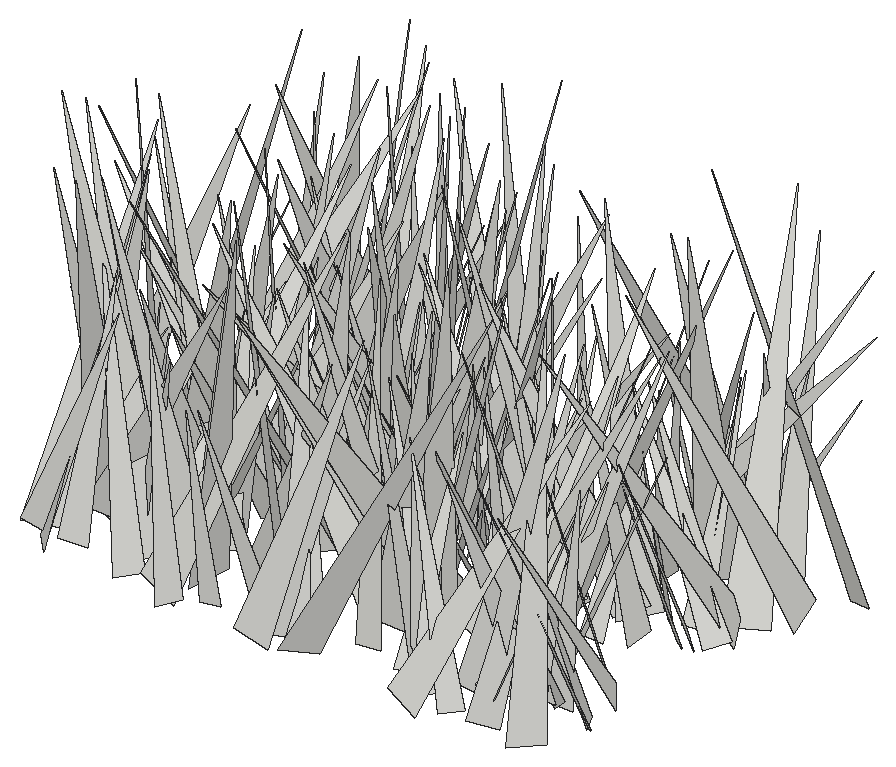
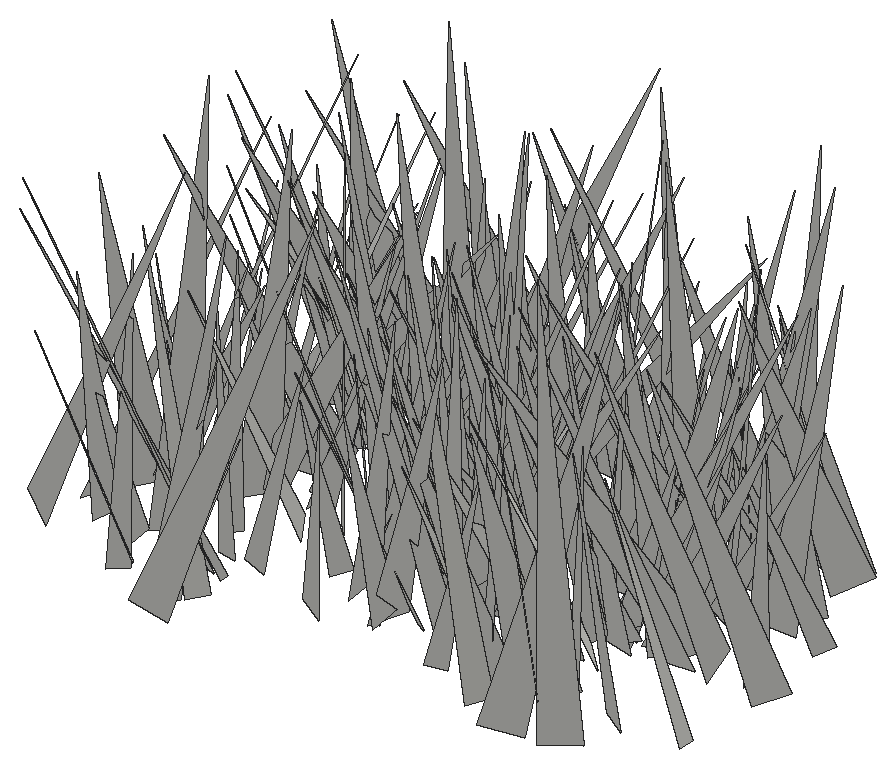
# SketchUp Ruby script. Lengths in inches.
U = 1.inch
M = Sketchup.active_model
def pt(a) = Geom::Point3d.new(a.map { |v| v * U })
def face(e, loops, mat)
  f = e.add_face(loops[0].map { |a| pt(a) })
  loops[1..].each { |l| e.add_face(l.map { |a| pt(a) }).erase! }
  f.material = f.back_material = mat if mat
  f
end
# faces: each face lists its corners as indices into pts; further lists are holes
def faces(e, pts, list, mat = nil) = list.each { |f| face(e, (f[0].is_a?(Array) ? f : [f]).map { |l| l.map { |i| pts[i] } }, mat) }
# xy, xz, yz: faces in a plane at the given z, y or x. An outline is a flat list of corners, or four numbers for a rectangle; further outlines are holes
def ring(l) = l.size == 4 ? [[l[0], l[1]], [l[2], l[1]], [l[2], l[3]], [l[0], l[3]]] : l.each_slice(2).to_a
def flat(e, list, mat, &to3) = list.each { |f| face(e, (f[0].is_a?(Array) ? f : [f]).map { |l| ring(l).map { |u, v| to3.(u, v) } }, mat) }
def xy(e, z, list, mat = nil) = flat(e, list, mat) { |x, y| [x, y, z] }
def xz(e, y, list, mat = nil) = flat(e, list, mat) { |x, z| [x, y, z] }
def yz(e, x, list, mat = nil) = flat(e, list, mat) { |y, z| [x, y, z] }
def lines(e, pts, list) = list.each { |a, b| e.add_line(pt(pts[a]), pt(pts[b])) }
# prism: a flat outline (further loops are holes) pulled along v
def prism(e, loops, v, mat = nil)
  f = face(e, loops, mat); d = Geom::Vector3d.new(v.map { |x| x * U })
  f.pushpull(f.normal.samedirection?(d) ? d.length : -d.length)
end
def box(e, o, s, mat = nil) = prism(e, [[o, [o[0] + s[0], o[1], o[2]], [o[0] + s[0], o[1] + s[1], o[2]], [o[0], o[1] + s[1], o[2]]]], [0, 0, s[2]], mat)
def at(x, y, z, deg = 0) = Geom::Transformation.translation(pt([x, y, z])) * Geom::Transformation.rotation(ORIGIN, Z_AXIS, deg.degrees)
def axes(o, x, y, z) = Geom::Transformation.new([*x, 0, *y, 0, *z, 0, *pt(o).to_a, 1])
def part(name) = M.definitions.add(name)
# library, detail: a bought-in or finely detailed component or shape, given as its bounding box
def library(name, o, s) = part(name).tap { |d| box(d.entities, o, s) }
def detail(e, o, s) = box(e.add_group.entities, o, s)
def put(e, d, t, mat = nil) = e.add_instance(d, t).tap { |i| i.material = mat if mat }
def group(e, t, mat = nil) = e.add_group.tap { |g| g.transformation = t; g.material = mat if mat }.entities
root = M.entities
c1 = part("fur_instance\#9")
p = [[0.8125,0,1.79],[0.67,-0.02,1.48],[0,-0.11,0],[0,0.11,0]]
faces(c1.entities,p,[[0,1,2,3]])
put(root,c1,axes([516.04,55.98,-21.66],[0.11042,6.13884,2.00494],[6.14565,0.51615,-1.91884],[1.98398,-1.94051,5.83229]))
put(root,c1,axes([512.14,56.45,-21.86],[-4.33048,1.8912,1.2808],[1.94847,4.49129,-0.04381],[1.19187,-0.47097,4.72523]))
put(root,c1,axes([515.34,57.75,-21.86],[0.25989,-4.12749,1.06746],[-4.12688,-0.51192,-0.97467],[-1.06982,0.97209,4.01917]))
put(root,c1,axes([513.26,57.27,-21.86],[0.17752,-3.57602,1.3313],[-3.7929,-0.31113,-0.32997],[-0.41733,1.30655,3.56518]))
put(root,c1,axes([524.42,56.25,-21.66],[-1.36293,4.52681,0.55653],[4.38086,1.13777,1.47406],[-1.26877,-0.93423,4.49185]))
put(root,c1,axes([512.15,58.58,-21.86],[7.47084,-2.00529,1.5784],[-1.88161,-7.62701,-0.78379],[-1.72397,-0.36551,7.69548]))
put(root,c1,axes([525.35,59.25,-21.66],[3.42862,-3.42654,1.21049],[-3.04602,-3.61734,-1.61199],[-1.98197,-0.36822,4.57144]))
put(root,c1,axes([505.53,57.5,-21.66],[1.80806,-4.3936,1.6396],[-4.55829,-1.23367,1.72079],[1.10181,2.10605,4.4285]))
put(root,c1,axes([522.51,55.97,-21.86],[1.42855,6.69806,0.59183],[6.31436,-1.12829,-2.47201],[2.31152,-1.05735,6.38701]))
put(root,c1,axes([528.0625,60.52,-21.66],[-4.13321,-3.41194,0.20507],[-3.07913,3.85633,2.10107],[1.48403,-1.5014,4.93054]))
put(root,c1,axes([520.01,61.89,-21.66],[4.91107,-6.51993,1.1851],[-5.42781,-4.80392,-3.93621],[-3.80168,-1.5638,7.15082]))
put(root,c1,axes([517.61,56.57,-21.86],[7.23014,-2.66142,0.8801],[-2.79977,-6.73645,2.62947],[0.1379,2.76941,7.24182]))
put(root,c1,axes([528.73,58.25,-21.66],[-3.23089,-3.2407,0.20186],[-3.09319,2.98531,-1.58167],[-0.98745,1.25194,4.29408]))
put(root,c1,axes([524.28,57.8,-21.66],[1.86303,-6.4471,2.90273],[-6.99316,-1.23765,1.73947],[1.04242,3.21946,6.48153]))
put(root,c1,axes([522.09,57.65,-21.86],[-5.84783,-0.54956,0.92386],[-0.66437,5.86496,-0.71656],[0.84507,0.80798,5.82972]))
put(root,c1,axes([527.625,56.3,-21.86],[-6.65914,2.85732,1.17721],[2.6023,6.69305,-1.52492],[1.66678,0.96593,7.084]))
put(root,c1,axes([507.0625,57.63,-21.86],[-0.99114,4.85366,1.48422],[5.00835,1.18049,-0.51592],[0.82303,-1.33855,4.92689]))
put(root,c1,axes([511.26,56.93,-21.86],[1.74287,7.71217,1.36191],[7.45298,-1.20484,-2.71503],[2.4053,-1.85492,7.42588]))
put(root,c1,axes([516.36,56.61,-21.66],[-3.94538,2.89092,1.6801],[2.22143,4.20848,-2.02488],[2.49909,0.82308,4.45234]))
put(root,c1,axes([511.22,59.15,-21.86],[-7.26017,0.65472,1.63239],[0.85,7.37598,0.82207],[1.53976,-0.9847,7.24313]))
put(root,c1,axes([505.85,61.03,-21.86],[7.57168,-2.77915,1.4038],[-2.39268,-7.55557,-2.05259],[-1.99233,-1.48808,7.80006]))
put(root,c1,axes([509.9,57.09,-21.86],[-5.44212,1.96061,0.21811],[1.90755,5.39324,-0.88463],[0.50284,0.7598,5.71648]))
put(root,c1,axes([522.05,57.79,-21.86],[-5.54219,0.95074,1.40051],[0.80502,5.69802,-0.68242],[1.48905,0.4581,5.58158]))
put(root,c1,axes([516.86,57.23,-21.86],[-0.46142,6.00885,1.03301],[6.04976,0.32253,0.82618],[-0.75742,-1.08443,5.96964]))
put(root,c1,axes([528.3,58.8,-21.86],[-5.87124,-3.56524,0.53214],[-3.58838,5.68376,-1.51131],[-0.34307,1.5651,6.70063]))
put(root,c1,axes([522.99,57.21,-21.86],[-1.18961,5.30841,0.21099],[4.92708,1.02155,2.07828],[-1.98686,-0.64508,5.02744]))
put(root,c1,axes([519.04,59.85,-21.86],[2.07554,-6.96607,1.71735],[-7.11885,-1.77704,1.39545],[0.89291,2.02467,7.13349]))
put(root,c1,axes([515.03,59.18,-21.86],[-6.35073,-3.49942,2.22612],[-3.7296,6.59945,-0.26567],[1.81428,1.31702,7.24617]))
put(root,c1,axes([526.82,59.08,-21.86],[-0.53957,3.97433,2.02364],[4.38519,0.84425,-0.48882],[0.81275,-1.91664,3.98089]))
put(root,c1,axes([506.27,56.99,-21.86],[5.15399,5.0376,1.12923],[4.93282,-5.27609,1.02292],[-1.5231,-0.04087,7.13405]))
put(root,c1,axes([516.63,58.53,-21.86],[-2.6188,2.85202,1.01974],[2.95253,2.70449,0.01846],[0.67563,-0.76402,3.87193]))
put(root,c1,axes([521.35,57.78,-21.86],[-2.23012,3.65012,0.738],[3.54975,2.34365,-0.86487],[1.12574,-0.15918,4.18913]))
put(root,c1,axes([506.74,59.58,-21.66],[3.69144,-5.31541,0.62902],[-5.0613,-3.21782,2.51095],[1.74141,1.9152,5.96452]))
put(root,c1,axes([508.74,59.09,-21.86],[2.33806,3.32528,1.40975],[3.5899,-2.32407,-0.47188],[-0.3968,-1.43269,4.03749]))
put(root,c1,axes([513.12,60.18,-21.86],[-0.06945,-5.66946,1.63507],[-5.27402,0.7929,2.5253],[2.64594,1.43164,5.07647]))
put(root,c1,axes([518.82,61.65,-21.66],[-6.06549,-1.51995,0.44377],[-1.27134,5.72216,2.22212],[0.94386,-2.06007,5.84487]))
put(root,c1,axes([508.1,60.32,-21.86],[-0.58442,-4.16845,1.10453],[-3.96593,0.95723,1.51414],[1.69333,0.80327,3.92746]))
put(root,c1,axes([526.97,58.9,-21.66],[-3.79929,-4.93063,0.76728],[-4.2284,2.66909,-3.78564],[-2.64961,2.81057,4.94112]))
put(root,c1,axes([519.73,60.25,-21.86],[-1.28539,6.13898,3.44989],[6.89976,0.39684,1.86462],[-1.40785,-3.66012,5.98853]))
put(root,c1,axes([519.67,61.17,-21.86],[3.37968,-7.43588,1.46776],[-7.57694,-3.27406,0.85991],[0.19143,1.6903,8.12251]))
put(root,c1,axes([519.47,57.99,-21.66],[1.15539,6.15443,1.22459],[6.01284,-1.44203,1.57415],[-1.79512,-0.86897,6.06086]))
put(root,c1,axes([517.6875,60.94,-21.86],[-6.93796,2.79801,1.11968],[3.01121,6.55067,2.28891],[0.12298,-2.54512,7.12215]))
put(root,c1,axes([508.34,60.32,-21.86],[-4.3642,6.37446,3.0679],[7.06974,4.05938,1.62241],[0.25406,-3.46117,7.553]))
put(root,c1,axes([527.34,61.21,-21.86],[-3.21192,-3.98216,0.77509],[-3.98629,3.28152,0.34045],[0.75355,0.38579,5.10471]))
put(root,c1,axes([525.59,56.5,-21.86],[-6.0414,2.82747,0.77084],[2.14541,5.47009,-3.25002],[1.99649,2.67784,5.82499]))
put(root,c1,axes([508.03,60.18,-21.86],[3.13173,2.6382,1.54856],[2.8558,-3.31576,-0.12654],[-1.0966,-1.10068,4.0929]))
put(root,c1,axes([517.27,60.86,-21.66],[-4.42248,-6.55022,0.11235],[-5.68971,3.77318,-3.9833],[-3.24733,2.30957,6.8262]))
put(root,c1,axes([505.37,60.8125,-21.86],[4.2743,-5.66959,1.70794],[-5.91958,-4.14155,1.06631],[-0.14077,2.00854,7.01974]))
put(root,c1,axes([509.79,62.02,-21.86],[3.73697,-5.4189,0.58942],[-5.45085,-3.71358,0.41766],[0.01126,0.72231,6.56925]))
put(root,c1,axes([508.87,62.68,-21.86],[4.42124,-3.27,0.9733],[-2.9097,-4.44582,-1.71927],[-1.78153,-0.85401,5.22344]))
put(root,c1,axes([509.76,58.5,-21.86],[-0.98442,7.82804,0.7856],[7.24103,0.59195,3.17514],[-3.07617,-1.11168,7.22258]))
put(root,c1,axes([522.64,59.99,-21.86],[4.59981,5.90875,0.46757],[5.722,-4.27232,-2.30133],[1.54616,-1.76752,7.12569]))
put(root,c1,axes([505.48,58.03,-21.86],[-5.30404,4.85737,1.41696],[4.30663,5.41145,-2.42976],[2.65607,0.92563,6.76928]))
put(root,c1,axes([505.62,61.94,-21.86],[0.65749,-6.30029,1.7132],[-6.47052,-0.85883,-0.67511],[-0.87239,1.62165,6.29842]))
put(root,c1,axes([516.83,60.64,-21.86],[2.82445,3.52777,0.66946],[3.53756,-2.58781,-1.2883],[0.61561,-1.31488,4.33162]))
put(root,c1,axes([508.14,62.72,-21.86],[3.30529,-7.09092,0.75642],[-7.06387,-3.14139,1.41833],[0.97724,1.27626,7.69379]))
put(root,c1,axes([511.31,63.19,-21.86],[0.9036,-5.03288,0.01557],[-4.93923,-0.88981,-0.97923],[-0.96652,-0.158,5.01871]))
put(root,c1,axes([516.96,61.66,-21.86],[-5.6933,-0.47947,0.5538],[-0.44449,5.71072,0.37467],[0.58224,-0.32872,5.70116]))
put(root,c1,axes([510.9,61.33,-21.86],[4.80209,-1.99507,1.20954],[-2.10711,-4.89697,0.2883],[-1.00169,0.73669,5.19204]))
put(root,c1,axes([524.43,61.03,-21.86],[0.51441,-3.71167,1.78135],[-3.92489,0.09986,1.3415],[1.24297,1.85145,3.49879]))
put(root,c1,axes([524.01,60.73,-21.66],[3.16186,-4.77933,2.12939],[-5.21892,-2.70344,1.68164],[0.37303,2.68757,5.47827]))
put(root,c1,axes([525.05,57.86,-21.66],[5.40862,3.75774,0.29196],[3.28966,-4.95573,2.84217],[-1.83956,2.18614,5.94103]))
put(root,c1,axes([524.74,60.17,-21.86],[2.40606,6.39383,1.08481],[6.38564,-2.13376,-1.58675],[1.13207,-1.55339,6.64473]))
put(root,c1,axes([506.83,59.79,-21.86],[1.15422,4.7345,0.08294],[4.6056,-1.10261,-1.15208],[1.10037,-0.35121,4.73502]))
put(root,c1,axes([510.72,60.25,-21.86],[4.79219,0.94532,0.41054],[0.81575,-4.67249,1.23678],[-0.62985,1.14081,4.72537]))
put(root,c1,axes([520.08,60.26,-21.86],[5.65388,1.0827,1.74004],[0.6959,-5.81697,1.3583],[-1.92762,1.07564,5.59407]))
put(root,c1,axes([507.53,62.72,-21.66],[-0.92246,-4.02488,0.49642],[-3.83236,0.69867,-1.45667],[-1.32631,0.78053,3.86377]))
put(root,c1,axes([513.9,62.4,-21.86],[5.17414,-4.36417,1.70527],[-4.54977,-5.28673,0.27499],[-1.1196,1.31532,6.76329]))
put(root,c1,axes([519.2,60.82,-21.86],[-1.66344,3.87519,0.54462],[3.91265,1.65754,0.1564],[0.06977,-0.56232,4.21422]))
put(root,c1,axes([522.48,62.14,-21.66],[4.18709,2.7222,0.51054],[2.74144,-3.94162,-1.4666],[0.39441,-1.502,4.77401]))
put(root,c1,axes([524.87,58.3,-21.66],[-5.0261,5.87636,0.71878],[5.2638,4.86732,-2.98524],[2.70938,1.44485,7.13314]))
put(root,c1,axes([521.29,62.61,-21.86],[-2.36065,-3.34559,0.0438],[-3.13879,2.19578,-1.44709],[-1.15883,0.86782,3.83035]))
put(root,c1,axes([503.47,62.08,-21.86],[2.74116,-2.85153,0.16279],[-2.64199,-2.44575,1.64616],[1.08517,1.2485,3.59657]))
put(root,c1,axes([508.52,60.76,-21.66],[-6.74078,-2.87477,2.26806],[-3.46071,6.55422,-1.97791],[1.19661,2.76122,7.05622]))
put(root,c1,axes([509.97,63,-21.86],[-3.40624,-2.616,1.08161],[-2.59295,3.56228,0.44999],[1.13575,0.28715,4.27123]))
put(root,c1,axes([511.57,60.17,-21.66],[-4.67511,2.29396,0.21165],[2.12082,4.47274,-1.63107],[0.89953,1.37696,4.94555]))
put(root,c1,axes([521.5,61.11,-21.86],[0.97735,4.73028,0.44464],[4.65378,-0.86171,-1.06216],[0.95682,-0.64061,4.71196]))
put(root,c1,axes([524.9,62.24,-21.86],[4.03846,2.29721,0.25382],[2.30928,-3.98992,-0.63131],[0.09403,-0.6739,4.60302]))
put(root,c1,axes([511.12,60.93,-21.86],[-0.71343,7.62578,1.29035],[7.14993,0.15622,3.02994],[-2.94889,-1.46615,7.03427]))
put(root,c1,axes([528.33,66.76,-21.66],[-6.95908,-3.88864,0.42907],[-3.38575,6.42493,3.31533],[1.96017,-2.70799,7.24975]))
put(root,c1,axes([513.23,67.33,-21.66],[-6.54697,-3.05595,0.68846],[-2.14459,5.53525,4.1758],[2.28332,-3.56338,5.89613]))
put(root,c1,axes([527.33,65.43,-21.86],[-2.98193,-4.15353,0.46379],[-3.81224,2.9367,1.78925],[1.71281,-0.69483,4.78981]))
put(root,c1,axes([510.08,64.82,-21.86],[-5.4355,-1.48683,0.1699],[-1.41481,5.31415,1.24191],[0.48767,-1.15472,5.49664]))
put(root,c1,axes([521.53,62.82,-21.86],[-4.34694,-0.07841,1.0456],[-0.20123,4.43859,-0.5037],[1.02905,0.53671,4.31837]))
put(root,c1,axes([516.125,64.84,-21.86],[-1.04012,-7.65192,1.88155],[-7.84849,1.17518,0.4406],[0.70237,1.80029,7.70971]))
put(root,c1,axes([509.3,60.47,-21.86],[-0.93463,7.10607,0.24964],[6.82555,0.96718,-1.97702],[1.99262,0.02006,6.88921]))
put(root,c1,axes([515.9,63.97,-21.86],[-2.53875,-3.10556,0.31926],[-3.0835,2.42999,-0.88252],[-0.48832,0.80145,3.91291]))
put(root,c1,axes([513.86,64.89,-21.86],[2.30675,-6.01681,0.97122],[-6.03702,-2.11321,1.24701],[0.83643,1.34116,6.32203]))
put(root,c1,axes([517.22,62.65,-21.86],[4.28943,0.41298,0.87796],[0.18379,-4.25331,1.1028],[-0.95267,1.03894,4.16576]))
put(root,c1,axes([515.67,67.39,-21.66],[-6.83742,-2.67371,1.15288],[-1.91772,6.34944,3.35188],[2.19094,-2.7864,6.53176]))
put(root,c1,axes([526.01,64.36,-21.86],[-5.16901,0.01394,1.37798],[0.15537,5.32107,0.52899],[1.36927,-0.55116,5.14189]))
put(root,c1,axes([509.5,62.41,-21.86],[-6.47288,0.26814,0.01301],[0.25719,6.28405,-1.55397],[0.07694,1.55212,6.2893]))
put(root,c1,axes([523.45,63.4,-21.86],[-5.82181,0.2065,0.70872],[0.14567,5.84473,-0.50632],[0.72368,0.48471,5.80343]))
put(root,c1,axes([513.8125,67.32,-21.66],[7.80685,-2.34529,0.78759],[-1.91376,-7.37702,-2.99744],[-1.56786,-2.67335,7.58041]))
put(root,c1,axes([516,62.43,-21.86],[4.21835,1.12148,1.8478],[0.48542,-4.44001,1.58659],[-2.10629,1.22277,4.06632]))
put(root,c1,axes([503.74,65.39,-21.86],[3.7269,-2.05729,0.24824],[-1.97365,-3.67974,-0.86491],[-0.63149,-0.64103,4.16823]))
put(root,c1,axes([523.16,64.53,-21.86],[-7.49054,-0.65717,0.9559],[-0.61994,7.54719,0.33069],[0.98046,-0.24861,7.51203]))
put(root,c1,axes([510.98,64.2,-21.86],[-4.32305,-4.69404,2.5219],[-5.10648,4.57733,-0.23372],[1.52244,2.02405,6.37716]))
put(root,c1,axes([509.55,65.57,-21.86],[-3.5976,-6.50533,0.64098],[-6.34012,3.29439,-2.15004],[-1.59153,1.58132,7.11613]))
put(root,c1,axes([518.57,65.36,-21.86],[2.79226,2.81825,2.22878],[3.51982,-2.71249,-0.9798],[-0.72174,-2.32521,3.84438]))
put(root,c1,axes([519.4375,62.07,-21.66],[5.08694,2.79276,1.06084],[2.31416,-5.00849,2.08845],[-1.88933,1.38471,5.41433]))
put(root,c1,axes([524.86,65.39,-21.66],[-3.6368,4.97548,2.15784],[5.29036,2.68314,2.72961],[-1.1932,-3.26854,5.52548]))
put(root,c1,axes([517.84,66.17,-21.86],[7.87771,-0.03675,0.30438],[0.03502,-7.66773,-1.83222],[-0.30459,-1.83219,7.66177]))
put(root,c1,axes([527.3,64.9,-21.86],[-2.96371,-3.18096,0.56073],[-3.21747,2.84043,-0.89238],[-0.28422,1.01488,4.25508]))
put(root,c1,axes([515.12,63.48,-21.86],[2.64419,5.03318,0.33977],[4.95036,-2.51506,-1.26831],[0.97076,-0.88412,5.54221]))
put(root,c1,axes([521.09,65.92,-21.66],[-4.22534,-4.50008,2.6097],[-4.33201,4.90527,1.44456],[2.88009,0.77613,6.00146]))
put(root,c1,axes([507.51,65.43,-21.86],[5.59181,-3.37862,1.09906],[-3.46581,-5.63815,0.30113],[-0.78177,0.82912,6.52631]))
put(root,c1,axes([524.73,63.37,-21.86],[-0.04754,4.40868,0.34675],[4.41199,0.07095,-0.29716],[0.30179,-0.34273,4.39891]))
put(root,c1,axes([516.64,65.86,-21.86],[3.42079,-7.2545,1.9343],[-7.49487,-3.17419,1.34998],[0.44283,2.31686,7.90614]))
put(root,c1,axes([523.89,62.34,-21.86],[7.63616,1.08232,1.22596],[0.61242,-7.3209,2.64853],[-1.51635,2.49367,7.24345]))
put(root,c1,axes([507.87,65.48,-21.86],[-4.20776,3.77593,1.0344],[3.85861,3.7428,2.0336],[-0.66241,-2.18328,5.27517]))
put(root,c1,axes([516.73,65.5,-21.86],[2.97768,-2.23657,0.59018],[-2.29034,-2.98547,0.24174],[-0.32391,0.5494,3.71623]))
put(root,c1,axes([515.92,64.9,-21.66],[-4.47703,-2.46915,0.00102],[-2.34184,4.24552,-1.62229],[-0.78262,1.42103,4.84857]))
put(root,c1,axes([514.94,63.19,-21.86],[-3.04551,1.64304,1.0176],[0.80196,2.80235,-2.12461],[1.7584,1.56764,2.73144]))
put(root,c1,axes([526.21,65.79,-21.86],[-2.56443,-3.19615,1.19823],[-3.34404,2.653,-0.08027],[0.6845,0.98675,4.09698]))
put(root,c1,axes([516.16,62,-21.86],[-7.01528,2.7432,0.95764],[2.14491,6.5776,-3.12905],[1.96,2.6204,6.85188]))
put(root,c1,axes([514.48,66.5,-21.86],[-0.63614,-4.28295,0.71253],[-4.25699,0.4736,-0.95381],[-0.85404,0.8295,4.22357]))
put(root,c1,axes([528.57,65.35,-21.66],[-2.74524,3.88345,0.46197],[3.73915,2.44095,1.70042],[-1.14601,-1.33847,4.4414]))
put(root,c1,axes([520.38,64.93,-21.66],[-2.56552,5.11443,0.44811],[4.78646,2.20153,2.27666],[-1.85689,-1.39139,5.24939]))
put(root,c1,axes([525.06,65.58,-21.86],[-6.40886,3.74132,2.19702],[3.96061,6.64492,0.23769],[1.77143,-1.32114,7.41717]))
put(root,c1,axes([528.2,66.07,-21.86],[-4.59292,1.38597,0.57425],[1.45174,4.5724,0.57548],[0.37836,-0.71958,4.76284]))
put(root,c1,axes([522.91,64.74,-21.66],[-0.96186,4.58475,0.31518],[4.19254,0.74357,1.97843],[-1.88199,-0.68675,4.24628]))
put(root,c1,axes([521.15,63.16,-21.66],[-7.41355,2.38035,1.13819],[1.92535,7.2016,-2.52036],[1.80404,2.09598,7.36713]))
put(root,c1,axes([520.15,64.08,-21.86],[-0.8094,5.47668,0.09308],[5.43232,0.79056,0.72297],[-0.70181,-0.19701,5.48875]))
put(root,c1,axes([509.26,65.52,-21.66],[-0.23432,4.6061,1.3303],[4.44797,-0.2882,1.78136],[-1.78924,-1.31967,4.25416]))
put(root,c1,axes([517.91,67.52,-21.66],[5.88193,4.68919,0.48239],[4.10623,-4.71789,-4.20698],[2.31519,-3.54559,6.23594]))
put(root,c1,axes([514.52,66.92,-21.86],[-4.6508,-5.63712,0.37429],[-5.36466,4.25457,-2.58191],[-1.77136,1.91537,6.83673]))
put(root,c1,axes([529.39,69.02,-21.86],[-7.29024,-1.74958,0.87658],[-1.40156,7.02793,2.37084],[1.36568,-2.12702,7.11251]))
put(root,c1,axes([514.15,66.66,-21.86],[-1.05055,-3.99645,1.56356],[-4.12582,0.49771,-1.49997],[-1.18067,1.81677,3.85037]))
put(root,c1,axes([515.91,66.29,-21.86],[0.25719,7.17904,2.90731],[6.91163,1.10018,-3.3281],[3.49578,-2.70337,6.36621]))
put(root,c1,axes([518.68,67.39,-21.86],[-5.33847,-0.05884,0.40473],[-0.0096,5.31499,0.64603],[0.40887,-0.64342,5.29956]))
put(root,c1,axes([524.11,68.13,-21.86],[4.60045,-1.39498,0.802],[-1.20201,-4.59424,-1.0961],[-1.06973,-0.83684,4.68067]))
put(root,c1,axes([508.78,65.98,-21.66],[0.50211,5.33526,1.29674],[5.04367,0.06639,-2.22613],[2.16978,-1.38897,4.87457]))
put(root,c1,axes([502.5625,66.07,-21.66],[4.48664,-4.30175,1.96808],[-4.72578,-3.95369,2.13158],[0.21294,2.89338,5.83878]))
put(root,c1,axes([516.06,65.4375,-21.66],[-6.64988,-1.58039,2.79885],[-2.32051,6.81074,-1.66765],[2.22405,2.38079,6.62853]))
put(root,c1,axes([509.01,66.19,-21.86],[1.78136,5.8506,1.71123],[6.09225,-1.76893,-0.29408],[-0.20572,-1.72409,6.10871]))
put(root,c1,axes([517.89,68.05,-21.86],[-3.47477,-5.64058,1.59223],[-5.83486,3.50381,-0.32112],[0.55295,1.52727,6.61718]))
put(root,c1,axes([527.04,66.1,-21.86],[-1.136,4.49998,0.83575],[4.53043,1.22799,-0.4539],[0.65076,-0.69355,4.61891]))
put(root,c1,axes([509.65,66.13,-21.66],[-4.5359,3.17744,2.60533],[2.766,5.23085,-1.56386],[3.0386,-0.01843,5.3127]))
put(root,c1,axes([525.61,69.3,-21.86],[4.47344,-6.57845,1.38646],[-6.62258,-4.59864,-0.45163],[-1.15746,0.88686,7.94253]))
put(root,c1,axes([526.44,67.37,-21.86],[4.12014,1.91723,1.34742],[2.03951,-4.27599,-0.15214],[-1.154,-0.71202,4.54182]))
put(root,c1,axes([512.42,67.23,-21.66],[-0.71726,5.0627,1.58469],[5.02661,0.13746,1.836],[-1.69568,-1.73401,4.77227]))
put(root,c1,axes([506.36,66.18,-21.66],[2.2285,7.10603,0.93052],[7.02267,-1.97084,-1.76797],[1.42959,-1.39565,7.23438]))
put(root,c1,axes([505.39,65.4,-21.66],[-6.44163,0.17845,3.84936],[-1.24896,6.99677,-2.4144],[3.64548,2.71245,5.9747]))
put(root,c1,axes([509.9375,67.65,-21.86],[2.9133,6.77269,2.26525],[7.08174,-2.424,-1.8604],[0.9217,-2.7826,7.13411]))
put(root,c1,axes([509.8,70.92,-21.86],[5.40513,-4.44008,1.03103],[-3.91993,-5.34397,-2.46351],[-2.32626,-1.31164,6.54682]))
put(root,c1,axes([515.21,67.09,-21.86],[-6.34859,-2.07949,3.15929],[-2.7531,6.77324,-1.07409],[2.59343,2.09974,6.59357]))
put(root,c1,axes([506.53,65.13,-21.66],[-2.61013,7.00123,1.33294],[6.01827,2.92557,-3.58165],[3.81765,0.17478,6.55758]))
put(root,c1,axes([514.9,66.85,-21.86],[5.61181,2.09612,1.30854],[1.89864,-5.73587,1.04566],[-1.58152,0.55181,5.89854]))
put(root,c1,axes([516.54,66.41,-21.86],[2.31766,5.02687,0.82298],[4.84651,-2.45447,1.34356],[-1.56781,-0.15629,5.3699]))
put(root,c1,axes([514.48,66.89,-21.66],[3.32895,2.2471,0.95718],[1.81279,-3.35751,1.57751],[-1.63691,0.85163,3.69362]))
put(root,c1,axes([515.55,67.02,-21.66],[1.80048,6.74236,1.9451],[6.61582,-2.30046,1.85022],[-2.33959,-1.31645,6.72888]))
put(root,c1,axes([512.46,66.67,-21.66],[4.4552,2.25801,0.37031],[2.04407,-4.29173,1.57715],[-1.02836,1.2518,4.7392]))
put(root,c1,axes([514.43,67.19,-21.86],[-5.96382,1.04535,0.88629],[0.82737,5.90096,-1.39268],[1.09259,1.23747,5.8924]))
put(root,c1,axes([519.47,67.99,-21.86],[-2.50227,2.59124,1.1484],[2.47228,2.74461,-0.80603],[1.38608,-0.21748,3.51087]))
put(root,c1,axes([522.22,66.67,-21.66],[4.78963,3.34115,0.62659],[3.09789,-4.73577,1.57225],[-1.39963,0.95165,5.62422]))
put(root,c1,axes([508.43,69.96,-21.86],[2.55754,-6.5759,0.86107],[-6.14173,-2.00015,2.96707],[2.50263,1.81158,6.40156]))
put(root,c1,axes([523.21,69.49,-21.86],[-1.15878,-4.12917,1.68532],[-4.31214,1.48176,0.66553],[1.13832,1.40977,4.23673]))
put(root,c1,axes([522.05,69.47,-21.86],[-1.05409,-4.02831,1.60299],[-4.27873,0.70037,-1.05356],[-0.69957,1.78611,4.02845]))
put(root,c1,axes([528.35,67.16,-21.86],[-5.32969,5.59283,1.04722],[5.46672,5.43108,-1.18331],[1.57839,0.07463,7.63447]))
put(root,c1,axes([503.14,69.94,-21.86],[4.64757,1.11707,0.03174],[1.0994,-4.54603,-0.98676],[0.20042,-0.96672,4.67697]))
put(root,c1,axes([516.54,69.68,-21.86],[3.53151,3.08583,1.68165],[3.37882,-3.63698,-0.42174],[-0.96639,-1.43941,4.67077]))
put(root,c1,axes([509.17,68.4,-21.86],[2.66286,4.62658,1.9724],[4.32664,-3.24515,1.77077],[-2.56433,-0.67099,5.03592]))
put(root,c1,axes([514.875,69.51,-21.66],[3.37481,3.69249,0.11879],[3.55193,-3.19874,-1.47981],[1.01606,-1.08238,4.77849]))
put(root,c1,axes([511.36,70.44,-21.86],[3.99412,4.65299,3.2629],[5.30006,-4.48907,-0.08624],[-2.05092,-2.53923,6.13155]))
put(root,c1,axes([508.5625,73.11,-21.86],[4.04445,-6.42376,0.8146],[-6.13253,-4.10829,-1.94934],[-2.07854,-0.37835,7.33638]))
put(root,c1,axes([514.43,68.76,-21.86],[7.1658,2.76652,1.69463],[2.58302,-7.35112,1.0785],[-1.96302,0.42601,7.60521]))
put(root,c1,axes([518.03,68.54,-21.66],[-7.28792,0.99409,0.70676],[0.80322,7.1337,-1.75122],[0.9179,1.65037,7.1439]))
put(root,c1,axes([509.48,67,-21.86],[4.44404,5.53922,0.27989],[5.13876,-4.2472,2.46279],[-2.08674,1.3376,6.66087]))
put(root,c1,axes([513.93,68.05,-21.66],[3.59429,3.23742,0.8797],[2.57384,-3.488,2.32011],[-2.15177,1.23558,4.24464]))
put(root,c1,axes([512.97,71.09,-21.86],[1.65267,-3.08975,1.39314],[-3.11179,-1.99748,-0.7386],[-1.34319,0.82596,3.42525]))
put(root,c1,axes([522.22,72.3,-21.86],[6.41369,-0.07562,0.05633],[-0.05586,-6.13403,-1.87481],[-0.07597,-1.87412,6.13403]))
put(root,c1,axes([525.53,72.43,-21.86],[5.23051,-1.10724,0.78196],[-0.81536,-5.06,-1.7109],[-1.08287,-1.53819,5.06527]))
put(root,c1,axes([530.3,70.84,-21.86],[-4.4516,-6.59475,1.62319],[-6.65602,3.85048,-2.61027],[-1.35017,2.76139,7.51625]))
put(root,c1,axes([522.13,70.99,-21.66],[4.7067,5.43888,0.18038],[4.50837,-3.76361,-4.15655],[3.04771,-2.83211,5.87006]))
put(root,c1,axes([510.15,72.25,-21.66],[7.393,0.04175,0.28729],[0.1077,-7.1937,-1.72622],[-0.26959,-1.72907,7.18877]))
put(root,c1,axes([525.42,69.71,-21.86],[-5.0928,-0.09663,0.30052],[-0.16718,4.94609,-1.24277],[0.26777,1.25023,4.93978]))
put(root,c1,axes([510.03,71.03,-21.86],[4.10331,-3.61689,0.17449],[-3.47529,-3.85943,1.7253],[1.0172,1.40442,5.19061]))
put(root,c1,axes([506.16,72.91,-21.66],[2.3597,-7.64104,0.82634],[-7.58316,-2.17409,1.55097],[1.25061,1.23463,7.84527]))
put(root,c1,axes([516.32,69.47,-21.86],[-6.63605,2.7216,0.19643],[2.70208,6.62626,-0.52374],[0.38006,0.41041,7.15332]))
put(root,c1,axes([522.77,70.92,-21.66],[5.32286,5.30667,0.20638],[4.93366,-4.8331,-2.97258],[1.96528,-2.23975,6.90343]))
put(root,c1,axes([526.34,70.25,-21.86],[3.78689,-0.0231,1.24793],[-0.32688,-3.86581,0.92039],[-1.20458,0.97644,3.67342]))
put(root,c1,axes([522.93,74.08,-21.86],[0.06912,-7.57158,0.2529],[-7.42195,-0.11839,-1.51598],[-1.51902,0.23392,7.41859]))
put(root,c1,axes([505.96,70.29,-21.86],[2.58353,5.00263,1.49189],[5.09313,-2.78069,0.50442],[-1.14546,-1.08079,5.60772]))
put(root,c1,axes([523.93,70.46,-21.66],[-3.59352,-1.36236,0.30323],[-1.35819,3.22059,-1.62619],[-0.32136,1.6227,3.48208]))
put(root,c1,axes([523.03,73.15,-21.86],[5.55902,-2.83125,1.90418],[-2.404,-5.83322,-1.65498],[-2.42129,-0.70867,6.01496]))
put(root,c1,axes([509.34,70.17,-21.86],[4.85297,5.01471,2.08252],[4.89411,-5.24941,1.23566],[-2.35199,-0.5761,6.86817]))
put(root,c1,axes([516.16,69.78,-21.66],[-5.21181,1.32812,1.31914],[0.83689,5.14396,-1.87252],[1.67442,1.56295,5.04188]))
put(root,c1,axes([510.93,68.76,-21.66],[-5.92228,3.52878,0.304],[3.26745,5.67188,-2.1844],[1.36692,1.73077,6.53866]))
put(root,c1,axes([527.9,69.85,-21.66],[-5.38629,2.97439,0.98855],[2.72826,5.41671,-1.43257],[1.54299,0.80541,5.98388]))
put(root,c1,axes([525.2,72.05,-21.66],[3.3764,2.66955,0.1135],[2.47122,-3.05035,-1.76859],[1.01611,-1.452,3.92412]))
put(root,c1,axes([518.71,70.6,-21.86],[1.26657,4.59176,1.22685],[4.36989,-1.62436,1.56816],[-1.86909,-0.68616,4.4977]))
